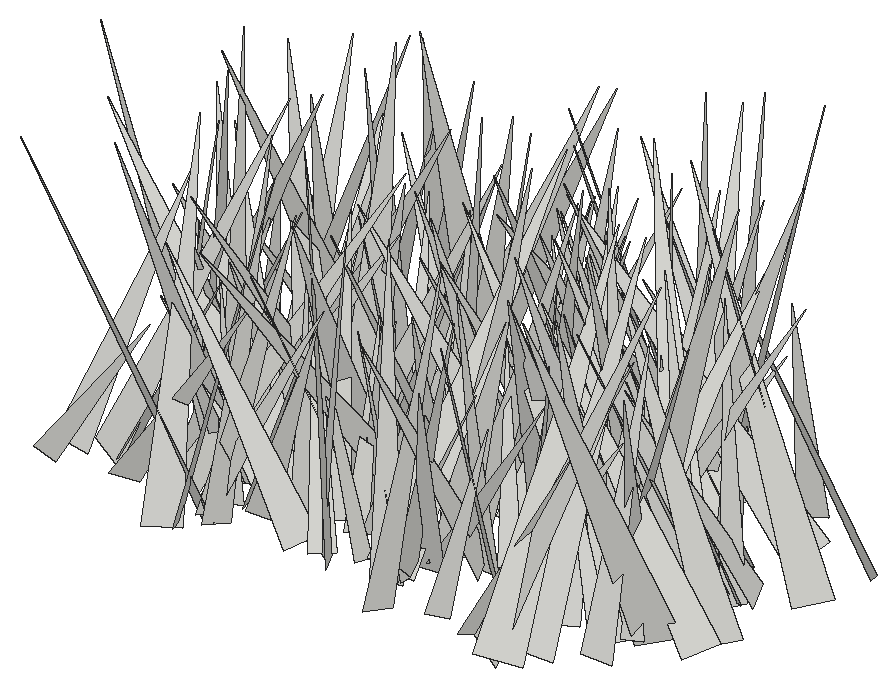
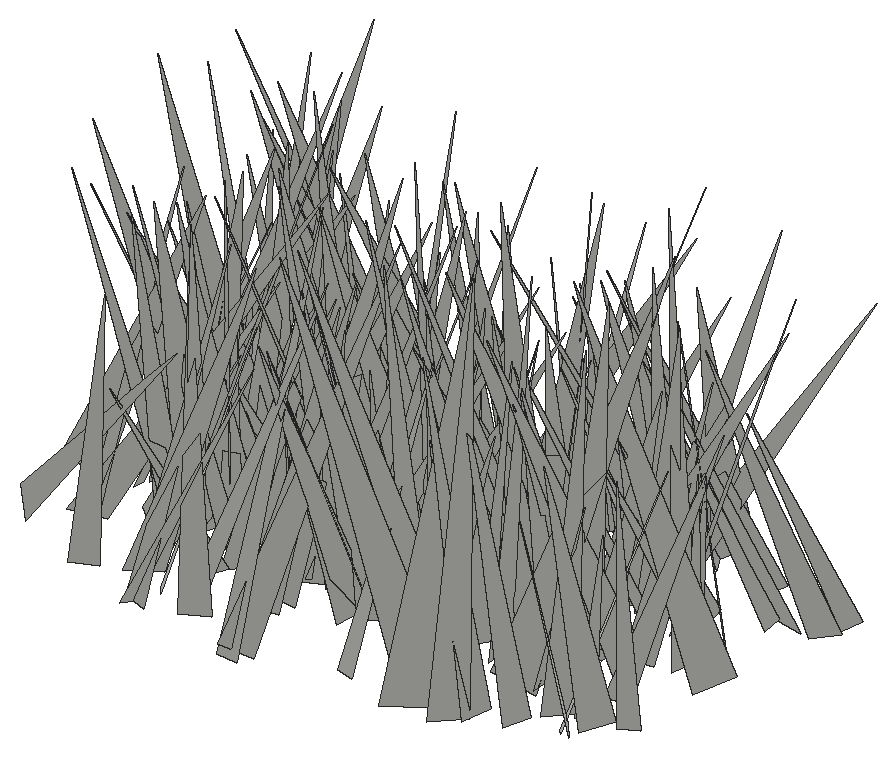
# SketchUp Ruby script. Lengths in inches.
U = 1.inch
M = Sketchup.active_model
def pt(a) = Geom::Point3d.new(a.map { |v| v * U })
def face(e, loops, mat)
  f = e.add_face(loops[0].map { |a| pt(a) })
  loops[1..].each { |l| e.add_face(l.map { |a| pt(a) }).erase! }
  f.material = f.back_material = mat if mat
  f
end
# faces: each face lists its corners as indices into pts; further lists are holes
def faces(e, pts, list, mat = nil) = list.each { |f| face(e, (f[0].is_a?(Array) ? f : [f]).map { |l| l.map { |i| pts[i] } }, mat) }
# xy, xz, yz: faces in a plane at the given z, y or x. An outline is a flat list of corners, or four numbers for a rectangle; further outlines are holes
def ring(l) = l.size == 4 ? [[l[0], l[1]], [l[2], l[1]], [l[2], l[3]], [l[0], l[3]]] : l.each_slice(2).to_a
def flat(e, list, mat, &to3) = list.each { |f| face(e, (f[0].is_a?(Array) ? f : [f]).map { |l| ring(l).map { |u, v| to3.(u, v) } }, mat) }
def xy(e, z, list, mat = nil) = flat(e, list, mat) { |x, y| [x, y, z] }
def xz(e, y, list, mat = nil) = flat(e, list, mat) { |x, z| [x, y, z] }
def yz(e, x, list, mat = nil) = flat(e, list, mat) { |y, z| [x, y, z] }
def lines(e, pts, list) = list.each { |a, b| e.add_line(pt(pts[a]), pt(pts[b])) }
# prism: a flat outline (further loops are holes) pulled along v
def prism(e, loops, v, mat = nil)
  f = face(e, loops, mat); d = Geom::Vector3d.new(v.map { |x| x * U })
  f.pushpull(f.normal.samedirection?(d) ? d.length : -d.length)
end
def box(e, o, s, mat = nil) = prism(e, [[o, [o[0] + s[0], o[1], o[2]], [o[0] + s[0], o[1] + s[1], o[2]], [o[0], o[1] + s[1], o[2]]]], [0, 0, s[2]], mat)
def at(x, y, z, deg = 0) = Geom::Transformation.translation(pt([x, y, z])) * Geom::Transformation.rotation(ORIGIN, Z_AXIS, deg.degrees)
def axes(o, x, y, z) = Geom::Transformation.new([*x, 0, *y, 0, *z, 0, *pt(o).to_a, 1])
def part(name) = M.definitions.add(name)
# library, detail: a bought-in or finely detailed component or shape, given as its bounding box
def library(name, o, s) = part(name).tap { |d| box(d.entities, o, s) }
def detail(e, o, s) = box(e.add_group.entities, o, s)
def put(e, d, t, mat = nil) = e.add_instance(d, t).tap { |i| i.material = mat if mat }
def group(e, t, mat = nil) = e.add_group.tap { |g| g.transformation = t; g.material = mat if mat }.entities
root = M.entities
c1 = part("fur_instance\#9")
p = [[0.8125,0,1.79],[0.67,-0.02,1.48],[0,-0.11,0],[0,0.11,0]]
faces(c1.entities,p,[[0,1,2,3]])
put(root,c1,axes([508.2,126.19,-21.86],[-4.67528,-5.85921,0.505],[-5.43274,4.05599,-3.23694],[-2.25181,2.37953,6.76097]))
put(root,c1,axes([518.74,128.69,-21.66],[-3.46675,-5.54657,1.13696],[-5.08588,3.63649,2.23277],[2.48816,-0.29493,6.14797]))
put(root,c1,axes([518.4,125.92,-21.86],[-1.839,3.01934,1.93742],[3.07994,2.44517,-0.88715],[1.83955,-1.07548,3.42218]))
put(root,c1,axes([511.83,126.73,-21.66],[-4.61226,3.61546,0.79034],[3.61757,4.1381,2.18138],[-0.78062,-2.18488,5.43931]))
put(root,c1,axes([516.79,124.68,-21.66],[-5.68198,1.58826,2.45655],[1.00817,6.10119,-1.61279],[2.74605,1.04639,5.67506]))
put(root,c1,axes([525.66,128.97,-21.66],[3.52912,-6.81057,1.30534],[-6.45742,-3.76145,-2.16695],[-2.52774,0.10047,7.35818]))
put(root,c1,axes([500.88,126.38,-21.86],[1.93678,-3.59499,0.72466],[-3.24209,-1.29543,2.2385],[1.71404,1.61186,3.41529]))
put(root,c1,axes([521.17,125.06,-21.86],[3.76818,7.24013,0.96766],[7.17608,-3.46602,-2.01138],[1.36373,-1.76699,7.91031]))
put(root,c1,axes([516.18,128.26,-21.86],[1.58205,-4.94043,0.08132],[-4.90313,-1.55912,0.66773],[0.6114,0.28046,5.1444]))
put(root,c1,axes([517.65,129.41,-21.66],[-5.63617,-2.55407,1.20627],[-1.85262,5.37498,2.72438],[2.13217,-2.08115,5.55585]))
put(root,c1,axes([520.44,125.45,-21.66],[6.21247,-1.9108,0.54363],[-1.98453,-5.88708,1.9863],[0.09123,2.05733,6.18874]))
put(root,c1,axes([504.27,126.5,-21.66],[3.95823,-3.37287,0.12226],[-3.1364,-3.60629,2.0534],[1.24667,1.63622,4.7778]))
put(root,c1,axes([516.01,127.05,-21.86],[5.74343,-0.59024,1.12729],[-0.57342,-5.85294,-0.14303],[-1.13593,-0.02976,5.77191]))
put(root,c1,axes([509.37,127.5625,-21.86],[2.31038,-4.41979,0.71264],[-4.3801,-2.06578,1.38834],[0.92579,1.25629,4.79008]))
put(root,c1,axes([507.76,126.71,-21.66],[2.74788,4.31889,0.7575],[4.17328,-2.30167,-2.01583],[1.34551,-1.68135,4.70533]))
put(root,c1,axes([522.2,124.5,-21.66],[-3.86216,7.0455,1.20437],[6.7899,4.04407,-1.88376],[2.2331,-0.11104,7.81068]))
put(root,c1,axes([507.36,129.03,-21.86],[-0.75565,-7.24529,1.23648],[-7.25287,0.53359,-1.30585],[-1.19119,1.34729,7.16659]))
put(root,c1,axes([507.19,124.9,-21.86],[-6.13848,3.83375,0.83292],[3.60337,6.1212,-1.61832],[1.55148,0.95163,7.05405]))
put(root,c1,axes([513.16,126.55,-21.86],[-6.29577,-3.22015,2.48262],[-3.79064,6.30377,-1.43636],[1.47099,2.46225,6.92409]))
put(root,c1,axes([508.2,126.38,-21.66],[5.34451,-1.51745,2.02584],[-2.07356,-5.33917,1.4711],[-1.45157,2.03988,5.35746]))
put(root,c1,axes([507.5,125.31,-21.86],[5.32876,3.34285,1.26399],[2.90072,-5.37113,1.97605],[-2.08763,1.0697,5.97207]))
put(root,c1,axes([515.55,126.69,-21.86],[-0.65155,5.99766,1.58433],[6.18323,0.49957,0.65163],[-0.49968,-1.63861,5.99765]))
put(root,c1,axes([520.91,126.85,-21.66],[0.51844,5.23573,1.343],[5.13497,-0.0558,-1.76472],[1.68777,-1.43851,4.95655]))
put(root,c1,axes([516.24,126.9,-21.66],[-4.21104,-1.2398,0.43934],[-1.31531,3.95873,-1.43574],[-0.00925,1.50143,4.14832]))
put(root,c1,axes([512.36,127.05,-21.86],[3.4021,4.35261,1.87369],[4.47593,-3.70904,0.48912],[-1.55627,-1.15238,5.50275]))
put(root,c1,axes([510.72,130.97,-21.86],[-3.43446,-5.67079,0.15135],[-5.3482,3.29577,2.1239],[1.89143,-0.97791,6.28032]))
put(root,c1,axes([514.88,128.17,-21.66],[3.85978,2.30102,0.3483],[2.28006,-3.60384,-1.45862],[0.46617,-1.42533,4.2503]))
put(root,c1,axes([511.56,126.99,-21.86],[-4.59387,1.36569,1.34916],[1.20913,4.77619,-0.71765],[1.49109,0.33451,4.73854]))
put(root,c1,axes([524.46,127.37,-21.86],[-3.36159,2.04077,0.19725],[2.04893,3.35754,0.1809],[0.07444,-0.25709,3.9284]))
put(root,c1,axes([513.67,131.35,-21.86],[2.28844,-6.77562,0.58153],[-5.77223,-2.2597,-3.61376],[-3.59563,-0.68473,6.17144]))
put(root,c1,axes([521.625,126.74,-21.86],[-5.36603,-1.88935,2.74168],[-2.67241,5.54565,-1.40882],[1.98613,2.35731,5.51173]))
put(root,c1,axes([522.54,125.79,-21.86],[-1.86477,7.56726,1.18834],[7.49142,2.05683,-1.34204],[1.5982,-0.81177,7.67722]))
put(root,c1,axes([522.85,129.71,-21.86],[2.01145,-6.31603,1.30369],[-6.40118,-2.12156,-0.40211],[-0.78536,1.11557,6.61638]))
put(root,c1,axes([508.73,125.93,-21.66],[-6.51752,1.2418,2.00991],[0.54856,6.53189,-2.25684],[2.29801,1.9627,6.23913]))
put(root,c1,axes([524.55,126.93,-21.86],[-0.07417,5.83715,1.21265],[5.95855,0.11247,-0.17697],[0.19614,-1.2097,5.83493]))
put(root,c1,axes([509.04,128.59,-21.66],[-3.24563,2.42896,0.17461],[2.25293,2.88449,1.75171],[-0.92447,-1.49811,3.65588]))
put(root,c1,axes([512.62,126.88,-21.86],[-3.8761,2.85036,0.12124],[2.83481,3.87102,-0.37744],[0.32105,0.23257,4.79648]))
put(root,c1,axes([519.66,128.32,-21.86],[1.13497,4.33314,1.68645],[4.04549,-0.06445,-2.557],[2.29221,-2.03177,3.67778]))
put(root,c1,axes([514.01,127.37,-21.86],[-4.83845,-0.36416,0.05457],[-0.36621,4.6838,-1.21411],[-0.03844,1.21473,4.69778]))
put(root,c1,axes([508.16,127.67,-21.86],[0.1057,3.9764,0.92499],[3.9126,-0.36287,1.11284],[-1.16573,-0.85739,3.81897]))
put(root,c1,axes([516.49,128.45,-21.66],[3.7348,-2.45498,0.02516],[-2.33086,-3.53122,1.44009],[0.77113,1.21649,4.23106]))
put(root,c1,axes([501.17,127.48,-21.86],[-0.64371,5.67181,1.6895],[5.48083,1.21245,-1.9821],[2.23257,-1.34117,5.35305]))
put(root,c1,axes([524.27,128.22,-21.86],[-2.23276,3.13779,0.67741],[3.20125,2.1153,0.75324],[-0.23799,-0.9847,3.77672]))
put(root,c1,axes([523.54,130.57,-21.86],[5.7747,-1.11479,0.95698],[-0.77258,-5.60537,-1.86777],[-1.24967,-1.68603,5.57685]))
put(root,c1,axes([503.08,128,-21.86],[4.1398,0.29454,0.02134],[0.28882,-4.10074,0.57065],[-0.06159,0.56772,4.11084]))
put(root,c1,axes([509.72,133.1,-21.66],[-6.50454,-4.83681,0.42708],[-4.2184,5.98256,3.50717],[2.40464,-2.5885,7.30777]))
put(root,c1,axes([508.45,127.96,-21.86],[4.19181,1.99584,0.5753],[1.88629,-4.2003,0.82769],[-0.86965,0.50967,4.56832]))
put(root,c1,axes([523.09,130.99,-21.66],[1.43067,-7.01564,1.7352],[-6.90944,-1.84641,-1.76845],[-2.11892,1.28394,6.9382]))
put(root,c1,axes([527.23,129.31,-21.66],[-4.14935,5.21761,0.66717],[4.85978,3.47746,3.02911],[-2.01273,-2.35998,5.93844]))
put(root,c1,axes([510.45,132.32,-21.66],[5.40488,-4.57462,0.50738],[-4.27322,-5.27816,-2.06831],[-1.71004,-1.26929,6.77215]))
put(root,c1,axes([517.88,129.37,-21.86],[-1.40726,-4.75955,2.034],[-5.17479,1.24906,-0.65748],[-0.10975,2.13481,4.91949]))
put(root,c1,axes([505.82,128.01,-21.86],[4.07618,6.66518,0.05677],[6.29765,-3.82934,-2.59208],[2.18344,-1.39809,7.37028]))
put(root,c1,axes([522.02,131.36,-21.66],[7.41722,0.99885,0.34739],[1.05742,-6.96886,-2.53978],[0.01548,-2.56338,7.04006]))
put(root,c1,axes([511.99,130.28,-21.86],[3.72524,-2.31212,0.81738],[-2.32656,-3.80205,-0.15146],[-0.77532,0.29988,4.38182]))
put(root,c1,axes([512.59,128.77,-21.86],[-2.95191,2.4359,0.97471],[2.3622,3.10602,-0.60836],[1.1418,-0.12828,3.77853]))
put(root,c1,axes([502.53,127.74,-21.86],[3.27574,7.01328,0.4286],[6.91428,-3.13335,-1.57325],[1.25002,-1.04703,7.57902]))
put(root,c1,axes([525.77,132.13,-21.86],[-4.47092,-4.93614,0.16266],[-4.90041,4.46105,0.68268],[0.61475,-0.33851,6.62484]))
put(root,c1,axes([525.66,131.81,-21.66],[-7.8024,0.71377,1.7229],[1.19599,7.6017,2.26696],[1.43089,-2.46171,7.49986]))
put(root,c1,axes([507.84,130.5,-21.66],[-6.653,2.83628,0.09553],[2.75112,6.38619,1.99099],[-0.69638,-1.86767,6.95291]))
put(root,c1,axes([506.9,129.8,-21.86],[-2.17172,3.54056,2.13295],[3.72846,2.71807,-0.7156],[1.78427,-1.37037,4.09143]))
put(root,c1,axes([522.53,132.44,-21.86],[7.53052,-1.13144,2.64431],[-0.30654,-7.68469,-2.41514],[-2.85982,-2.15562,7.22191]))
put(root,c1,axes([505.82,129.68,-21.86],[-7.70081,-2.50661,0.76749],[-2.60656,7.57519,-1.4131],[0.27927,1.58364,7.97425]))
put(root,c1,axes([511.45,128.96,-21.86],[3.60121,-2.60608,3.3834],[-3.59297,-4.24118,0.55747],[-2.30861,2.53545,4.41017]))
put(root,c1,axes([524.2,129.78,-21.86],[-3.20539,-1.99252,1.2784],[-2.28309,3.17085,-0.78241],[0.62603,1.36182,3.69222]))
put(root,c1,axes([515.37,127.19,-21.66],[-1.37451,8.097,0.63904],[7.82187,1.49419,-2.10823],[2.18815,-0.25501,7.93763]))
put(root,c1,axes([527.21,130.5,-21.86],[-3.75455,5.21199,1.89568],[5.51913,3.28609,1.89629],[-0.5456,-2.62523,6.13723]))
put(root,c1,axes([524.68,128.34,-21.66],[-0.02832,7.80203,1.3013],[7.5934,-0.33756,2.1891],[-2.2148,-1.25708,7.48868]))
put(root,c1,axes([507.48,128.3,-21.66],[-7.86516,0.65945,1.92725],[0.13584,7.83978,-2.12819],[2.03241,2.02799,7.60042]))
put(root,c1,axes([516.28,129.33,-21.86],[6.87844,-2.02965,2.77665],[-2.6588,-7.07628,1.41394],[-2.18175,2.22463,7.03088]))
put(root,c1,axes([503.32,130.24,-21.86],[4.60486,4.04407,1.88978],[4.30358,-4.74303,-0.33665],[-1.18533,-1.50984,6.1193]))
put(root,c1,axes([505.51,132.22,-21.86],[-0.2394,-4.99537,0.47277],[-5.01072,0.21306,-0.28607],[-0.26442,0.48521,4.99291]))
put(root,c1,axes([521.96,127.97,-21.86],[-5.97227,4.9002,0.90124],[4.6479,5.98621,-1.7477],[1.79477,0.80344,7.52499]))
put(root,c1,axes([503.59,132.1,-21.86],[7.9282,0.66664,2.15118],[1.11346,-8.00329,-1.62351],[-1.9576,-1.85234,7.78877]))
put(root,c1,axes([506.97,132.64,-21.86],[3.23703,-3.40023,0.62778],[-3.13183,-3.24768,-1.44163],[-1.46538,-0.57015,4.46784]))
put(root,c1,axes([504.95,132.84,-21.86],[3.29812,-3.00828,0.87507],[-2.53709,-3.30998,-1.81667],[-1.83812,-0.82908,4.07763]))
put(root,c1,axes([513.32,132.52,-21.86],[1.53045,-4.60076,0.23907],[-4.60681,-1.52625,0.11946],[0.03806,0.26453,4.84716]))
put(root,c1,axes([515.41,131.52,-21.66],[-2.41735,-5.08882,0.8159],[-4.81582,1.90935,-2.35956],[-1.83565,1.69223,5.11586]))
put(root,c1,axes([506.5625,129.95,-21.86],[-3.46559,5.8146,1.30946],[5.95968,3.40104,0.67057],[0.08042,-1.46897,6.73574]))
put(root,c1,axes([518.24,130.09,-21.86],[-1.47936,3.73163,0.54523],[3.76451,1.42617,0.45319],[-0.22551,-0.67216,3.98851]))
put(root,c1,axes([520.37,131.61,-21.86],[-3.06281,-3.15709,1.43812],[-3.29391,3.24851,0.11628],[1.08883,0.94666,4.3971]))
put(root,c1,axes([519.88,134.1,-21.86],[-0.91329,-6.82842,0.06821],[-6.63421,0.90353,1.6239],[1.61843,-0.14959,6.69511]))
put(root,c1,axes([504.88,129.0625,-21.86],[4.59265,0.40937,1.72839],[-0.43371,-4.3881,2.19176],[-1.72245,2.19644,4.05662]))
put(root,c1,axes([518.02,131.99,-21.86],[7.89082,-0.9052,1.78608],[-0.78265,-8.07818,-0.63641],[-1.84308,-0.44515,7.91703]))
put(root,c1,axes([508.69,129.45,-21.66],[-2.09774,5.99421,0.07606],[5.73274,1.98235,1.88224],[-1.75272,-0.69034,6.06533]))
put(root,c1,axes([505.8,131,-21.86],[3.2036,5.15972,0.63397],[4.7617,-2.61371,-2.78969],[2.08586,-1.95793,5.39475]))
put(root,c1,axes([523.96,131.15,-21.86],[-1.38179,3.78074,1.32931],[4.00762,1.30133,0.46468],[-0.00636,-1.40818,3.99842]))
put(root,c1,axes([504.28,130.7,-21.86],[0.5553,3.90242,1.15183],[3.90207,-0.84018,0.96535],[-1.15302,-0.96393,3.8217]))
put(root,c1,axes([509.94,131.73,-21.86],[1.20072,-3.47995,0.99765],[-3.52529,-0.88496,1.15597],[0.82322,1.28603,3.49507]))
put(root,c1,axes([504.01,131.14,-21.86],[0.50374,3.60666,1.32904],[3.78488,-0.69911,0.46265],[-0.67011,-1.23747,3.61216]))
put(root,c1,axes([520.93,132.04,-21.86],[-6.43604,2.78332,0.65453],[2.85741,6.20344,1.71766],[-0.1023,-1.83529,6.79846]))
put(root,c1,axes([516.53,134.28,-21.86],[6.011,-2.52803,0.45147],[-2.2406,-5.7244,-2.22212],[-1.25478,-1.8887,6.13068]))
put(root,c1,axes([515.65,133.47,-21.66],[3.87648,-5.20572,1.47803],[-5.00062,-4.14086,-1.46909],[-2.0683,0.2548,6.32205]))
put(root,c1,axes([526.08,133.85,-21.86],[-4.91943,-1.92287,0.32626],[-1.70701,4.67316,1.80343],[0.9434,-1.57124,4.96446]))
put(root,c1,axes([518.125,134.2,-21.86],[4.34994,-4.04005,0.73934],[-3.73736,-4.34022,-1.72779],[-1.70317,-0.79441,5.67968]))
put(root,c1,axes([516.08,130.6,-21.66],[6.10707,-2.19869,2.10682],[-2.76305,-5.98564,1.76265],[-1.28003,2.43046,6.24689]))
put(root,c1,axes([513.16,128.97,-21.86],[5.49101,0.89671,2.25711],[-0.37206,-5.20349,2.97239],[-2.40004,2.85822,4.70322]))
put(root,c1,axes([522.17,131.875,-21.66],[6.94828,-4.27135,1.74082],[-4.55894,-6.83788,1.41876],[-0.70067,2.13364,8.03182]))
put(root,c1,axes([516.23,133.62,-21.66],[-6.42762,0.7775,0.36666],[0.8533,6.10569,2.01137],[0.10407,-2.04186,6.15412]))
put(root,c1,axes([516.34,129.82,-21.86],[-6.72177,-1.11045,3.37602],[-2.29516,6.87097,-2.30972],[2.71346,3.06096,6.4094]))
put(root,c1,axes([517.19,135.23,-21.86],[-6.3203,-1.31951,1.76492],[-0.3807,5.93404,3.07318],[2.17051,-2.80147,5.67828]))
put(root,c1,axes([503.69,130.92,-21.86],[4.45385,0.90104,0.34779],[0.77968,-4.32278,1.21461],[-0.57002,1.12752,4.37874]))
put(root,c1,axes([509.72,131.89,-21.86],[3.41975,6.53108,1.33927],[6.45057,-2.86091,-2.51965],[1.68487,-2.30293,6.92828]))
put(root,c1,axes([515.78,135.11,-21.86],[-5.24067,-3.21189,0.67738],[-2.84495,5.08085,2.08111],[1.63749,-1.45206,5.78359]))
put(root,c1,axes([526.13,132.71,-21.66],[-3.48224,-3.77241,0.29956],[-3.58403,3.15695,-1.90663],[-1.21472,1.49981,4.76674]))
put(root,c1,axes([513.63,133.18,-21.86],[-3.32783,-6.52848,3.29816],[-6.89122,4.01297,0.99019],[2.45153,2.41834,7.26051]))
put(root,c1,axes([501.76,132.77,-21.66],[6.68383,-3.60485,0.36068],[-3.59385,-6.50181,1.61538],[0.45749,1.59067,7.42019]))
put(root,c1,axes([510.86,133.77,-21.86],[-3.91635,-3.27614,1.36892],[-3.24396,4.13005,0.60351],[1.44353,0.39293,5.07017]))
put(root,c1,axes([513.86,132.37,-21.86],[4.3952,-2.19196,2.60814],[-2.70598,-4.83259,0.49862],[-2.06997,1.6632,4.88608]))
put(root,c1,axes([515.35,133.74,-21.86],[3.09975,-1.98369,0.33098],[-1.98147,-3.11644,-0.1208],[-0.34401,0.07615,3.67817]))
put(root,c1,axes([514.55,131.4,-21.66],[0.6459,3.9486,0.07217],[3.68247,-0.62859,1.43463],[-1.42692,0.16515,3.73504]))
put(root,c1,axes([509.28,133.02,-21.86],[-5.12716,5.45276,3.67809],[5.84452,5.9162,-0.62364],[3.01704,-2.19425,7.45865]))
put(root,c1,axes([522.25,130.96,-21.66],[-1.13308,6.40977,0.66119],[6.08836,1.28481,-2.02171],[2.11049,-0.26515,6.18722]))
put(root,c1,axes([524.69,132.09,-21.86],[-5.52094,1.92393,0.48296],[1.85996,5.5174,-0.71721],[0.68943,0.52184,5.80241]))
put(root,c1,axes([503.7,135.69,-21.66],[3.91388,-2.85851,1.41513],[-2.09693,-3.9939,-2.26798],[-2.40345,-1.17037,4.2832]))
put(root,c1,axes([522.04,133.2,-21.86],[5.84499,-0.86217,1.83487],[-1.09003,-6.05756,0.62599],[-1.70936,0.91471,5.87498]))
put(root,c1,axes([505.78,133.3,-21.66],[5.9864,-4.39629,0.74457],[-4.35138,-5.48795,2.58196],[0.97326,2.50473,6.96403]))
put(root,c1,axes([508.09,134.6,-21.86],[3.45559,-4.90486,0.92565],[-4.98413,-3.32981,0.96246],[0.2699,1.30779,5.9222]))
put(root,c1,axes([510.24,133.65,-21.86],[6.4862,-0.82849,0.61771],[-0.87391,-6.49276,0.46816],[-0.55158,0.54452,6.52212]))
put(root,c1,axes([522.33,136.6,-21.66],[-7.22673,-3.69522,1.05519],[-3.3656,7.17065,2.06111],[1.85494,-1.38592,7.85061]))
put(root,c1,axes([516.13,132.54,-21.86],[-0.30009,3.62925,0.24074],[3.53668,0.34756,-0.831],[0.84929,-0.16496,3.54556]))
put(root,c1,axes([507.43,136.7,-21.86],[0.76231,-8.24421,0.75454],[-8.09051,-0.90251,-1.68715],[-1.75496,0.57958,8.10565]))
put(root,c1,axes([525.88,132.73,-21.86],[-5.20641,1.3754,0.94823],[1.21962,5.25029,-0.91901],[1.14166,0.66356,5.30602]))
put(root,c1,axes([524.38,132.23,-21.86],[-4.81407,6.51041,0.79127],[6.55623,4.75265,0.78417],[-0.16528,-1.10168,8.05889]))
put(root,c1,axes([506.42,133.04,-21.86],[1.48764,5.46016,1.29529],[5.56167,-1.25605,-1.09283],[0.74757,-1.52092,5.55267]))
put(root,c1,axes([521.42,132.35,-21.86],[1.31333,6.20143,0.89],[6.24264,-1.21867,-0.72041],[0.52849,-1.01577,6.2979]))
put(root,c1,axes([521.2,133.54,-21.66],[4.19059,5.13354,0.34706],[4.85008,-3.79176,-2.47669],[1.71767,-1.81771,6.14657]))
put(root,c1,axes([506.77,134,-21.86],[-4.39266,5.33205,2.64396],[5.82364,4.52851,0.54275],[1.2274,-2.40386,6.88706]))
put(root,c1,axes([517.49,137.13,-21.86],[-0.22294,-7.81188,0.28991],[-7.80547,0.20653,-0.4373],[-0.42917,0.30182,7.80282]))
put(root,c1,axes([515.375,133.01,-21.86],[-3.03856,4.16793,1.35783],[3.96538,3.31773,-1.3102],[1.86846,-0.26309,4.98878]))
put(root,c1,axes([520.87,135.45,-21.86],[2.48728,-3.44318,0.65298],[-3.47724,-2.52444,-0.0662],[-0.43662,0.49004,4.24707]))
put(root,c1,axes([519.91,134.625,-21.86],[-1.21907,-3.82959,1.50139],[-4.09681,0.98993,-0.80143],[-0.36895,1.66143,3.93822]))
put(root,c1,axes([507.74,132.09,-21.86],[-3.21539,5.33291,0.27404],[5.21793,3.20577,-1.16191],[1.13501,0.36996,6.11789]))
put(root,c1,axes([525.96,136.79,-21.66],[-7.44265,2.94787,0.75024],[2.95668,6.54484,3.6151],[-0.71474,-3.62229,7.14241]))
put(root,c1,axes([509.06,135.37,-21.86],[-6.68895,-1.28776,2.75903],[-1.15,7.23488,0.5888],[2.81923,-0.10417,6.78629]))
put(root,c1,axes([510.78,134.04,-21.86],[-5.92753,-0.80933,1.51712],[-1.07571,5.99367,-1.00549],[1.34146,1.2301,5.89742]))
put(root,c1,axes([521.63,134.53,-21.86],[4.46233,4.90899,2.88894],[5.22756,-4.98695,0.39938],[-2.26203,-1.84084,6.62202]))
put(root,c1,axes([524.53,135.375,-21.86],[-2.45002,-3.17903,0.27674],[-3.09062,2.27713,-1.20338],[-0.79426,0.94543,3.82893]))
put(root,c1,axes([515.06,134.49,-21.66],[5.08074,5.57509,0.64514],[5.46993,-4.72427,-2.25231],[1.25607,-1.97773,7.19879]))
put(root,c1,axes([506.59,135.31,-21.86],[3.71133,-3.4553,1.19556],[-3.62183,-3.7076,0.52772],[-0.50083,1.20708,5.04327]))
put(root,c1,axes([521.76,134.35,-21.66],[6.06814,-4.77445,2.10475],[-5.2154,-5.64781,2.22478],[-0.15808,3.05854,7.39379]))
put(root,c1,axes([516.98,135.43,-21.86],[2.55776,-3.86723,2.22173],[-4.13899,-3.01226,-0.47827],[-1.66143,1.55064,4.61182]))
put(root,c1,axes([521.24,134.23,-21.86],[-3.21117,5.73542,2.2751],[5.803,3.67883,-1.08356],[2.09673,-1.39782,6.48325]))
put(root,c1,axes([520.82,135.57,-21.86],[-0.87207,-5.64239,2.10409],[-5.67136,0.05471,-2.20385],[-2.02471,2.277,5.26688]))
put(root,c1,axes([519.84,136.36,-21.86],[-5.01187,1.13995,1.85475],[1.60842,5.07616,1.22637],[1.46717,-1.67079,4.99142]))
put(root,c1,axes([513.82,135.4,-21.86],[5.2265,3.38981,1.10604],[3.55749,-5.09026,-1.20993],[-0.2416,-1.62138,6.11091]))
put(root,c1,axes([528.15,134.29,-21.66],[-2.68904,7.46116,1.26428],[7.06219,1.99214,3.26422],[-2.71897,-2.20471,7.22805]))
put(root,c1,axes([515.9,135.43,-21.86],[1.63751,6.97927,2.94123],[7.53115,-1.18196,-1.38823],[0.80173,-3.15202,7.03309]))
put(root,c1,axes([512.11,137.14,-21.66],[-5.24413,-0.63684,1.6828],[-0.10679,5.28634,1.66778],[1.7961,-1.54509,5.01248]))
put(root,c1,axes([519,134.22,-21.86],[1.83922,3.08635,0.93557],[2.6886,-2.06216,1.51739],[-1.78108,0.07419,3.25666]))
put(root,c1,axes([525.78,136.88,-21.86],[-4.39451,-5.32367,1.29551],[-5.40377,4.48556,0.10243],[0.905,0.93264,6.90237]))
put(root,c1,axes([504.96,133.38,-21.86],[7.28027,0.47928,1.68125],[-0.05604,-7.13268,2.27604],[-1.74733,2.22571,6.93193]))
put(root,c1,axes([518.52,135.92,-21.86],[0.21554,-5.31829,2.18174],[-5.56977,-0.73327,-1.23719],[-1.42193,2.0661,5.17688]))
put(root,c1,axes([504.09,138.32,-21.86],[-3.67716,-3.23058,0.06887],[-2.92053,3.36739,2.02339],[1.38271,-1.47883,4.45691]))
put(root,c1,axes([517.43,138.05,-21.86],[2.94915,-5.28887,0.70098],[-5.06545,-3.02722,-1.5291],[-1.67475,-0.15728,5.85931]))
put(root,c1,axes([502.37,136.72,-21.86],[0.87128,-4.23502,0.75689],[-4.24446,-0.72019,0.85631],[0.702,0.90186,4.23807]))
put(root,c1,axes([512.32,137.19,-21.86],[-1.91573,-3.10975,0.18965],[-3.07242,1.92263,0.49017],[0.51647,-0.09744,3.61944]))
put(root,c1,axes([504.83,137.43,-21.86],[5.63565,-3.00774,1.4531],[-2.80235,-5.80815,-1.15361],[-1.81792,-0.37081,6.28301]))
put(root,c1,axes([506.59,136.25,-21.86],[-3.7389,-0.44853,0.79303],[-0.43438,3.82202,0.11371],[0.80087,-0.02096,3.764]))
put(root,c1,axes([520.51,135.68,-21.66],[2.74298,6.25055,1.8619],[6.47418,-2.36552,-1.59662],[0.78801,-2.32269,6.63657]))
put(root,c1,axes([514.06,136.31,-21.86],[0.68635,-5.64905,2.27441],[-5.90756,-0.06201,1.6287],[1.47832,2.3749,5.45254]))
put(root,c1,axes([515.26,134.99,-21.86],[3.32598,3.77438,0.4675],[3.78797,-3.34308,0.04133],[-0.34022,-0.32329,5.03054]))
put(root,c1,axes([509.96,135.03,-21.86],[-3.18277,2.93848,0.48438],[2.88307,3.21784,-0.5768],[0.74643,0.10079,4.29324]))
put(root,c1,axes([523.46,133.58,-21.86],[-6.0602,5.67803,0.65626],[5.53411,6.06799,-1.39639],[1.4298,0.57987,8.18634]))
put(root,c1,axes([516,141.14,-21.66],[6.60243,-3.6292,1.16999],[-2.40466,-5.77841,-4.35427],[-2.95933,-3.40161,6.14845]))
put(root,c1,axes([510.49,137.86,-21.66],[0.32033,-6.88611,1.90206],[-6.92731,0.16595,1.76741],[1.74605,1.92169,6.66313]))
put(root,c1,axes([514.65,136.59,-21.86],[4.92372,-1.23429,0.65682],[-1.32256,-4.89156,0.72207],[-0.45359,0.86432,5.02445]))
put(root,c1,axes([503.88,137.22,-21.86],[0.6335,-3.36408,1.34348],[-3.58683,-0.77327,-0.24494],[-0.50657,1.2682,3.41444]))
put(root,c1,axes([520.88,139.15,-21.86],[-3.83157,-3.11067,0.41222],[-2.87249,3.73899,1.51524],[1.26294,-0.9332,4.69694]))
put(root,c1,axes([514.61,136.23,-21.66],[4.76351,-2.22786,1.63166],[-2.67424,-4.53288,1.61806],[-0.68857,2.19233,5.00362]))
put(root,c1,axes([512.34,139.77,-21.86],[-2.61623,-5.06997,0.16776],[-4.93297,2.58676,1.24576],[1.18261,-0.42604,5.56752]))
put(root,c1,axes([522.16,135.51,-21.66],[-7.61718,0.0241,1.98426],[-0.51537,7.57673,-2.07045],[1.91631,2.1335,7.33043]))
put(root,c1,axes([510.59,137.36,-21.86],[-3.73959,3.61146,1.09906],[3.77498,3.58144,1.07604],[0.00944,-1.53809,5.08619]))
put(root,c1,axes([523.87,134.87,-21.86],[-7.99125,0.08509,2.25297],[-0.74491,7.73167,-2.93422],[2.12796,3.02611,7.43355]))
put(root,c1,axes([509.57,137.35,-21.86],[1.82991,-7.19945,3.13467],[-7.38413,-0.48301,3.20126],[2.67073,3.59742,6.70317]))
put(root,c1,axes([519.91,137.07,-21.66],[0.48143,3.7055,0.846],[3.27794,0.02687,-1.98307],[1.92393,-0.97302,3.16701]))
put(root,c1,axes([522.75,135.76,-21.66],[7.20277,3.49638,1.97973],[3.12762,-7.42996,1.74287],[-2.5223,0.77133,7.81454]))
put(root,c1,axes([521.09,140.3,-21.86],[-2.89154,-5.8907,0.51675],[-5.81601,2.937,0.93617],[1.06836,0.04534,6.49499]))
put(root,c1,axes([528.4,137.28,-21.86],[-4.35257,-4.39527,0.35538],[-3.69396,3.36161,-3.66659],[-2.40819,2.78761,4.98191]))
put(root,c1,axes([516.18,141.4,-21.86],[-3.49524,-7.20934,0.56433],[-6.86604,3.50524,2.25399],[2.26947,-0.49846,7.68835]))
put(root,c1,axes([505.65,138.72,-21.86],[5.71322,-0.96407,0.62556],[-0.92485,-5.73993,-0.39936],[-0.68221,-0.29224,5.7802]))
put(root,c1,axes([509.35,140.29,-21.86],[6.25935,-4.83068,2.00086],[-4.50057,-6.56633,-1.77386],[-2.66155,-0.25726,7.70509]))
put(root,c1,axes([519.71,138.68,-21.86],[-4.9951,-5.23204,0.99068],[-5.30492,4.77148,-1.54841],[-0.46216,1.77916,7.06595]))
put(root,c1,axes([507.36,140.33,-21.66],[7.0973,-2.99001,1.53723],[-2.6894,-7.20395,-1.59536],[-2.01752,-0.91535,7.53436]))
put(root,c1,axes([521.97,138.71,-21.66],[-5.92654,3.46188,1.28835],[3.68281,5.72588,1.55549],[0.28525,-1.99951,6.68498]))
put(root,c1,axes([524.11,139.3125,-21.86],[2.34766,-4.1804,1.05082],[-4.25289,-2.44131,-0.21062],[-0.70205,0.80976,4.78987]))
put(root,c1,axes([518.91,139.74,-21.86],[1.30695,-5.86281,0.96642],[-5.89292,-1.15208,0.98022],[0.76158,1.14664,5.9262]))
put(root,c1,axes([503.91,138.08,-21.86],[3.13745,2.7412,0.96065],[2.81213,-3.22064,0.00574],[-0.7273,-0.62763,4.16626]))
put(root,c1,axes([503.3,137.27,-21.86],[-4.2045,3.84796,1.64776],[3.68267,4.51063,-1.13666],[1.98995,-0.21727,5.58504]))
put(root,c1,axes([521.26,140.45,-21.86],[-4.78281,-0.5343,0.54387],[-0.29464,4.48183,1.81189],[0.70318,-1.75621,4.45846]))
put(root,c1,axes([507.03,139.21,-21.86],[6.44965,-0.53992,1.19924],[-0.48241,-6.55498,-0.35669],[-1.22351,-0.26161,6.46237]))
put(root,c1,axes([509.24,139.26,-21.66],[5.85705,-5.48153,0.51052],[-5.36351,-5.5136,2.33363],[1.24121,2.04104,7.67505]))
